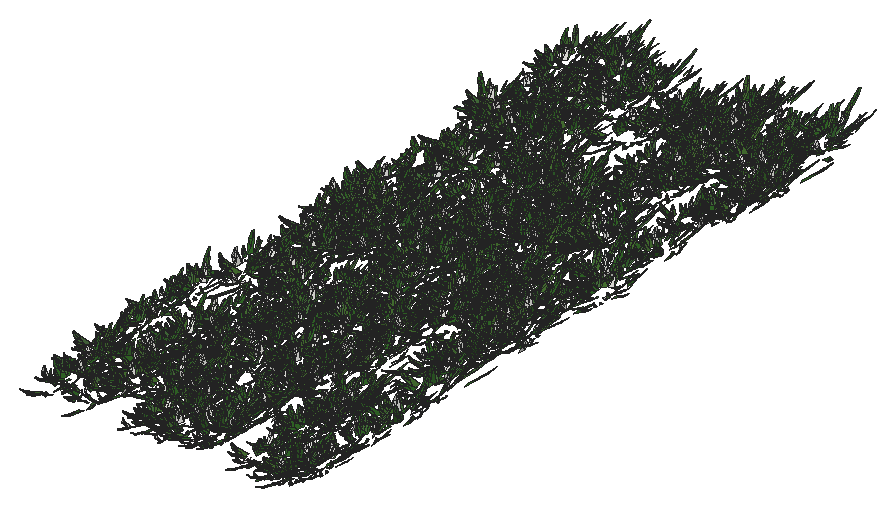
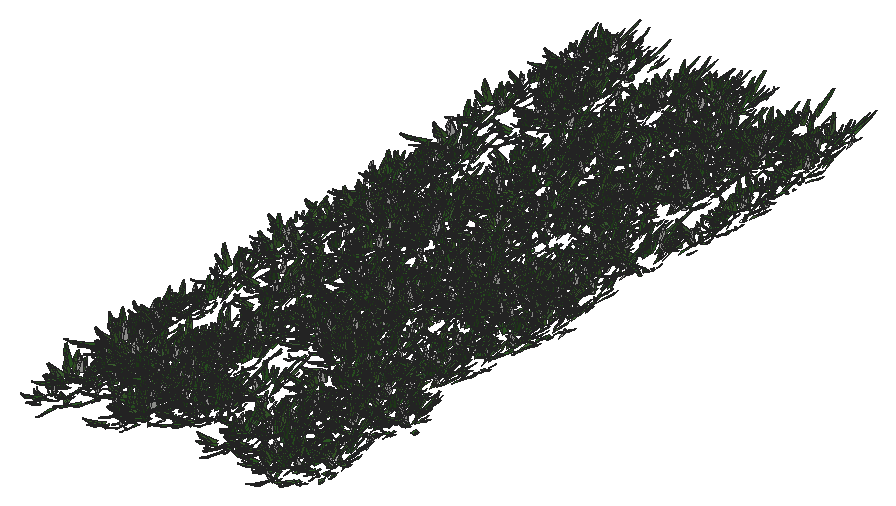
# SketchUp Ruby script. Lengths in inches.
U = 1.inch
M = Sketchup.active_model
def pt(a) = Geom::Point3d.new(a.map { |v| v * U })
def face(e, loops, mat)
  f = e.add_face(loops[0].map { |a| pt(a) })
  loops[1..].each { |l| e.add_face(l.map { |a| pt(a) }).erase! }
  f.material = f.back_material = mat if mat
  f
end
# faces: each face lists its corners as indices into pts; further lists are holes
def faces(e, pts, list, mat = nil) = list.each { |f| face(e, (f[0].is_a?(Array) ? f : [f]).map { |l| l.map { |i| pts[i] } }, mat) }
# xy, xz, yz: faces in a plane at the given z, y or x. An outline is a flat list of corners, or four numbers for a rectangle; further outlines are holes
def ring(l) = l.size == 4 ? [[l[0], l[1]], [l[2], l[1]], [l[2], l[3]], [l[0], l[3]]] : l.each_slice(2).to_a
def flat(e, list, mat, &to3) = list.each { |f| face(e, (f[0].is_a?(Array) ? f : [f]).map { |l| ring(l).map { |u, v| to3.(u, v) } }, mat) }
def xy(e, z, list, mat = nil) = flat(e, list, mat) { |x, y| [x, y, z] }
def xz(e, y, list, mat = nil) = flat(e, list, mat) { |x, z| [x, y, z] }
def yz(e, x, list, mat = nil) = flat(e, list, mat) { |y, z| [x, y, z] }
def lines(e, pts, list) = list.each { |a, b| e.add_line(pt(pts[a]), pt(pts[b])) }
# prism: a flat outline (further loops are holes) pulled along v
def prism(e, loops, v, mat = nil)
  f = face(e, loops, mat); d = Geom::Vector3d.new(v.map { |x| x * U })
  f.pushpull(f.normal.samedirection?(d) ? d.length : -d.length)
end
def box(e, o, s, mat = nil) = prism(e, [[o, [o[0] + s[0], o[1], o[2]], [o[0] + s[0], o[1] + s[1], o[2]], [o[0], o[1] + s[1], o[2]]]], [0, 0, s[2]], mat)
def at(x, y, z, deg = 0) = Geom::Transformation.translation(pt([x, y, z])) * Geom::Transformation.rotation(ORIGIN, Z_AXIS, deg.degrees)
def axes(o, x, y, z) = Geom::Transformation.new([*x, 0, *y, 0, *z, 0, *pt(o).to_a, 1])
def part(name) = M.definitions.add(name)
# library, detail: a bought-in or finely detailed component or shape, given as its bounding box
def library(name, o, s) = part(name).tap { |d| box(d.entities, o, s) }
def detail(e, o, s) = box(e.add_group.entities, o, s)
def put(e, d, t, mat = nil) = e.add_instance(d, t).tap { |i| i.material = mat if mat }
def group(e, t, mat = nil) = e.add_group.tap { |g| g.transformation = t; g.material = mat if mat }.entities
root = M.entities
M.materials.add("Material10").color = [48, 90, 38]
M.materials.add("Material11").color = [68, 110, 48]
M.materials.add("Material12").color = [48, 90, 48]
M.materials.add("Material13").color = [58, 110, 58]
M.materials.add("Material14").color = [58, 90, 38]
M.materials.add("Material15").color = [68, 100, 58]
M.materials.add("Material16").color = [48, 100, 38]
M.materials.add("Material9").color = [68, 110, 58]
c1 = part("grass00")
p = [[-0.6875,0.15,0],[-0.56,0.08,5.52],[-0.04,0.03,2.76],[0.48,-0.02,0],[0.35,-0.02,5.52],[-0.1,-0.14,5.52],
  [-0.12,0.65,8.37],[-0.42,0.65,8.37]]
faces(c1.entities,p,[[0,1,2,3],[3,2,4],[1,5,2],[5,4,2],[1,6,5],[4,5,6],[7,6,1]])
c2 = part("Group16\#1")
put(c2.entities,c1,axes([1.44,-0.61,-0.01],[0.05352,0.12609,0],[-0.10704,0.04543,0.07239],[0.06664,-0.02828,0.11628]),"Material12")
put(c2.entities,c1,axes([0.76,-0.15,-0.01],[0.04676,0.24062,0],[-0.23162,0.04501,0.06642],[0.0652,-0.01267,0.23595]),"Material9")
put(c2.entities,c1,axes([0.79,0.01,-0.01],[-0.00606,0.34651,0],[-0.34381,-0.00602,0.0432],[0.04319,0.00076,0.34386]))
put(c2.entities,c1,axes([1,0.23,-0.01],[-0.07192,0.31144,0],[-0.28722,-0.06632,0.1236],[0.12043,0.02781,0.29478]),"Material11")
put(c2.entities,c1,axes([1.66,0.77,-0.01],[-0.13828,0.29651,0],[-0.21551,-0.1005,0.22471],[0.20365,0.09498,0.23779]),"Material16")
put(c2.entities,c1,axes([0.6875,0.52,-0.01],[-0.18126,0.24051,0],[-0.22746,-0.17142,0.09788],[0.07817,0.05891,0.28481]),"Material11")
put(c2.entities,c1,axes([0.68,0.78,-0.01],[-0.215,0.18688,0],[-0.12385,-0.14248,0.21334],[0.13995,0.16101,0.18878]),"Material9")
put(c2.entities,c1,axes([0.56,1,-0.01],[-0.13756,0.07624,0],[-0.06159,-0.11112,0.0927],[0.04494,0.08108,0.12705]),"Material11")
put(c2.entities,c1,axes([0.2,0.64,-0.01],[-0.23729,0.07254,0],[-0.05711,-0.18681,0.153],[0.04473,0.14632,0.19535]),"Material16")
put(c2.entities,c1,axes([0.0625,0.72,-0.01],[-0.28874,0.02525,0],[-0.02179,-0.24916,0.14647],[0.01276,0.14591,0.25012]),"Material9")
put(c2.entities,c1,axes([-0.08,0.62,-0.01],[-0.34089,-0.04187,0],[0.03255,-0.26504,0.216],[-0.02633,0.21439,0.26703]),"Material16")
put(c2.entities,c1,axes([-0.34,0.98,-0.01],[-0.14314,-0.0493,0],[0.04397,-0.12769,0.06843],[-0.02228,0.0647,0.13505]),"Material16")
put(c2.entities,c1,axes([-0.87,1.45,-0.01],[-0.23488,-0.14114,0],[0.13761,-0.22901,0.06087],[-0.03135,0.05217,0.26717]))
put(c2.entities,c1,axes([-0.72,0.77,-0.01],[-0.14208,-0.13251,0],[0.07209,-0.0773,0.16301],[-0.11118,0.11922,0.1057]),"Material16")
put(c2.entities,c1,axes([-0.62,0.43,-0.01],[-0.14845,-0.21203,0],[0.18654,-0.13061,0.12304],[-0.10079,0.07057,0.22772]),"Material9")
put(c2.entities,c1,axes([-0.68,0.29,-0.01],[-0.13639,-0.32136,0],[0.31723,-0.13464,0.05579],[-0.05136,0.0218,0.34462]),"Material10")
put(c2.entities,c1,axes([-0.64,0.125,-0.01],[-0.0458,-0.23569,0],[0.22124,-0.043,0.08276],[-0.08124,0.01579,0.22538]),"Material13")
put(c2.entities,c1,axes([-1.6,-0.03,-0.01],[0.00576,-0.32897,0],[0.27526,0.00482,0.18018],[-0.18015,-0.00315,0.2753]),"Material11")
put(c2.entities,c1,axes([-1.36,-0.31,-0.01],[0.05718,-0.24765,0],[0.18172,0.04196,0.17267],[-0.16825,-0.03885,0.1865]),"Material16")
put(c2.entities,c1,axes([-1.54,-0.72,-0.01],[0.06537,-0.14017,0],[0.13555,0.06321,0.03939],[-0.0357,-0.01665,0.14956]))
put(c2.entities,c1,axes([-1.19,-0.9,-0.01],[0.09597,-0.12735,0],[0.11214,0.08451,0.07557],[-0.06035,-0.04548,0.14042]),"Material15")
put(c2.entities,c1,axes([-0.47,-0.54,-0.01],[0.11588,-0.10072,0],[0.0618,0.0711,0.12124],[-0.07953,-0.0915,0.0942]))
put(c2.entities,c1,axes([-0.47,-0.84,-0.01],[0.11927,-0.0661,0],[0.06603,0.11913,0.00646],[-0.00313,-0.00565,0.13621]),"Material11")
put(c2.entities,c1,axes([-0.38,-1.24,-0.01],[0.28037,-0.08571,0],[0.0618,0.20215,0.20315],[-0.05939,-0.19428,0.21139]),"Material15")
put(c2.entities,c1,axes([-0.06,-0.66,-0.01],[0.22719,-0.01987,0],[0.01247,0.14255,0.17758],[-0.01547,-0.17691,0.1431]),"Material14")
put(c2.entities,c1,axes([0.11,-0.89,-0.01],[0.14882,0.01828,0],[-0.01058,0.08611,0.12229],[0.01491,-0.12138,0.08676]),"Material12")
put(c2.entities,c1,axes([0.25,-0.72,-0.01],[0.20481,0.07053,0],[-0.06206,0.18022,0.10291],[0.03351,-0.0973,0.1906]),"Material12")
put(c2.entities,c1,axes([0.85,-1.42,-0.01],[0.16481,0.09904,0],[-0.09472,0.15762,0.05616],[0.02893,-0.04814,0.18389]),"Material11")
put(c2.entities,c1,axes([1.01,-1.09,-0.01],[0.21858,0.20385,0],[-0.17495,0.1876,0.15339],[0.10462,-0.11218,0.25652]),"Material16")
put(c2.entities,c1,axes([1.01,-0.71,-0.01],[0.08733,0.12473,0],[-0.06445,0.04512,0.13037],[0.1068,-0.07477,0.07867]),"Material12")
c3 = part("Group15\#1")
put(c3.entities,c2,at(0,0,0))
c4 = part("3darcstudiotree_grass00\#1")
put(c4.entities,c3,at(0,0,0))
put(root,c4,axes([889.11,700.2,12.99],[-2.48857,4.83217,0],[-1.60041,-4.30668,-0.00331],[-0.00933,-0.0251,1.47415]))
put(root,c4,axes([889.45,555.4,12.99],[1.88325,-5.62415,0],[2.2145,3.87465,-0.00025],[0.00077,0.00134,1.45509]))
put(root,c4,axes([890.7,736.79,12.99],[-0.67721,-6.67786,0],[3.30552,-1.75159,-0.01344],[0.04021,-0.02131,1.42931]))
put(root,c4,axes([890.59,527.43,12.99],[1.23508,-6.86534,0],[2.79631,2.62859,-0.00107],[0.00335,0.00315,1.41133]))
put(root,c4,axes([890.07,729.8,12.99],[-1.4659,5.84935,0],[-2.43711,-3.19136,-0.00674],[-0.02223,-0.02911,1.46389]))
put(root,c4,axes([890.29,569.96,12.99],[-1.20792,5.92922,0],[-2.43583,-2.59295,-0.01596],[-0.07323,-0.07796,1.86544]))
put(root,c4,axes([890.73,542.65,12.99],[1.71513,4.00539,0],[-2.12111,4.74593,-0.01876],[-0.05829,0.13042,1.77063]))
put(root,c4,axes([890.87,639.05,12.99],[1.25364,6.64692,0],[-3.14878,3.10311,-0.01792],[-0.0469,0.04622,1.34035]))
put(root,c4,axes([892.5,617.87,12.99],[1.99351,-5.07033,0],[1.82805,3.75557,-0.01288],[0.04404,0.09047,1.54961]))
put(root,c4,axes([893.14,588.73,12.99],[-2.84145,-1.64891,0],[0.79806,-7.18594,-0.00944],[0.0101,-0.09094,1.93444]))
put(root,c4,axes([894.38,665.36,12.99],[-2.41994,-3.76289,0],[1.7496,-5.87931,-0.01911],[0.03346,-0.11243,1.32815]))
put(root,c4,axes([894.17,700.75,12.99],[-2.72326,-0.10093,0],[0.04495,-6.33677,-0.00434],[0.00025,-0.03592,1.37632]))
put(root,c4,axes([894.41,648.52,12.99],[-2.77624,2.98667,0],[-1.27115,-6.17405,-0.0027],[-0.00443,-0.02152,1.57765]))
put(root,c4,axes([894.45,517.39,12.99],[1.92472,-5.7589,0],[2.22303,3.88219,-0.00592],[0.02191,0.03827,1.78738]))
put(root,c4,axes([894.51,633.23,12.99],[-0.10576,6.13122,0],[-3.20045,-0.28845,-0.01193],[-0.05367,-0.00484,1.97773]))
put(root,c4,axes([894.76,507.46,12.99],[0.73477,5.96043,0],[-2.82287,1.81831,-0.02067],[-0.08381,0.05398,1.69495]))
put(root,c4,axes([895.09,711.14,12.99],[2.7201,4.30897,0],[-1.8665,6.15665,-0.01195],[-0.02082,0.06867,1.37528]))
put(root,c4,axes([897.43,681,12.99],[-3.04265,0.35823,0],[-0.15997,-7.0997,-0.00589],[-0.00096,-0.04283,1.35922]))
put(root,c4,axes([898.1,740.56,12.99],[0.23179,-7.22579,0],[2.54694,0.4269,-0.00239],[0.00971,0.00163,1.42634]))
put(root,c4,axes([897,605.72,12.99],[0.62032,6.83292,0],[-2.78217,1.31977,-0.00381],[-0.01551,0.00736,1.62105]))
put(root,c4,axes([898.29,717.4,12.99],[0.42937,-6.32449,0],[2.49768,0.88604,-0.00401],[0.02082,0.00739,1.82024]))
put(root,c4,axes([898.53,618.78,12.99],[0.91628,-5.1494,0],[2.52826,2.35071,-0.0011],[0.00494,0.0046,1.80895]))
put(root,c4,axes([899.48,673.55,12.99],[2.62988,-0.99399,0],[0.55692,7.69933,-0.01648],[0.00872,0.1206,1.51991]))
put(root,c4,axes([899.46,586.64,12.99],[3.4134,1.62353,0],[-0.71308,7.83371,-0.01168],[-0.00692,0.07599,1.39591]))
put(root,c4,axes([900.61,741.23,12.99],[3.44408,-0.25415,0],[0.08694,6.15631,-0.01793],[0.00281,0.19875,1.79317]))
put(root,c4,axes([901.875,703.72,12.99],[0.0032,-6.22666,0],[2.78842,0.0075,-0.01884],[0.07166,0.00019,1.45492]))
put(root,c4,axes([902.12,635.8,12.99],[-2.06596,5.7417,0],[-2.57655,-4.84423,-0.01702],[-0.05495,-0.10332,1.91367]))
put(root,c4,axes([902.1,525.17,12.99],[3.06635,-0.29682,0],[0.12679,6.84401,-0.02002],[0.00349,0.18854,1.69539]))
put(root,c4,axes([903.61,693.23,12.99],[-3.37213,2.17513,0],[-0.90079,-7.29706,-0.00145],[-0.00158,-0.01283,1.8291]))
put(root,c4,axes([903.07,617.46,12.99],[0.95242,7.49428,0],[-2.36141,1.5681,-0.00931],[-0.03611,0.02398,1.3628]))
put(root,c4,axes([904.85,656.18,12.99],[-2.23753,5.4106,0],[-2.13955,-4.62327,-0.01805],[-0.05563,-0.12022,1.71251]))
put(root,c4,axes([905.1875,628.21,12.99],[-2.35532,2.72791,0],[-1.18826,-5.3609,-0.00642],[-0.01064,-0.04801,1.3229]))
put(root,c4,axes([905.07,670.3125,12.99],[-1.67258,4.18596,0],[-2.56199,-5.34901,-0.00484],[-0.0117,-0.02443,1.55938]))
put(root,c4,axes([906.18,644.99,12.99],[-0.78923,-5.50789,0],[3.27099,-2.44906,-0.01545],[0.0482,-0.03609,1.54954]))
put(root,c4,axes([906.22,508.02,12.99],[-0.37406,-5.96975,0],[3.38961,-1.10978,-0.00214],[0.00721,-0.00236,1.59988]))
put(root,c4,axes([905.29,591.09,12.99],[-1.61058,4.76543,0],[-2.42445,-4.28152,-0.01374],[-0.04386,-0.07746,1.69563]))
put(root,c4,axes([905.04,544.16,12.99],[-0.8341,7.12764,0],[-3.0028,-1.83613,-0.00132],[-0.00556,-0.0034,1.858]))
put(root,c4,axes([904.75,618.24,12.99],[2.4007,5.25585,0],[-2.3435,5.59327,-0.01961],[-0.04836,0.11543,1.65716]))
put(root,c4,axes([906.12,532.9,12.99],[-2.70473,0.752,0],[-0.41791,-7.85407,-0.00408],[-0.00182,-0.03415,1.74968]))
put(root,c4,axes([905.07,714.26,12.99],[0.47893,7.6528,0],[-3.19759,1.04564,-0.02596],[-0.07693,0.02516,1.32635]))
put(root,c4,axes([905.23,633.26,12.99],[-0.79693,7.39381,0],[-3.19145,-1.79739,-0.00818],[-0.03214,-0.0181,1.82396]))
put(root,c4,axes([906.84,736.01,12.99],[-2.61883,4.34404,0],[-1.63817,-5.16033,-0.01293],[-0.03819,-0.12029,1.92389]))
put(root,c4,axes([905.92,605.375,12.99],[2.18903,5.14094,0],[-2.299,5.11509,-0.004],[-0.01232,0.02742,1.89371]))
put(root,c4,axes([907.25,563.7,12.99],[-3.06581,1.10697,0],[-0.44175,-6.39285,-0.01239],[-0.00708,-0.10252,1.42361]))
put(root,c4,axes([906.32,552.57,12.99],[3.11337,0.63617,0],[-0.24083,6.15863,-0.01038],[-0.00483,0.12358,1.94021]))
put(root,c4,axes([907.1,694.13,12.99],[1.37515,5.77822,0],[-2.19205,2.7259,-0.01685],[-0.0837,0.10408,1.93576]))
put(root,c4,axes([909.91,733.37,12.99],[-2.98753,-4.03038,0],[1.29962,-5.03369,-0.01139],[0.02516,-0.09747,1.52439]))
put(root,c4,axes([910,522.94,12.99],[-0.33669,-7.20196,0],[2.55571,-0.62431,-0.01446],[0.06571,-0.01605,1.61179]))
put(root,c4,axes([909.59,517.17,12.99],[-2.31485,3.45016,0],[-1.62215,-5.68696,-0.02083],[-0.04485,-0.15725,1.60618]))
put(root,c4,axes([910.25,718.3,12.99],[-2.81133,-1.91296,0],[0.82005,-6.29725,-0.0137],[0.01382,-0.10615,1.39479]))
put(root,c4,axes([910.65,618.72,12.99],[2.31372,-3.04681,0],[1.57401,6.24565,-0.00508],[0.00919,0.03648,1.56982]))
put(root,c4,axes([911.38,580.73,12.99],[1.12741,-7.37052,0],[2.72279,2.17621,-0.01723],[0.05902,0.04717,1.43549]))
put(root,c4,axes([911.67,587.49,12.99],[-2.23921,5.74187,0],[-2.01313,-4.10222,-0.02096],[-0.07106,-0.14481,1.6805]))
put(root,c4,axes([911.47,701.26,12.99],[0.50465,7.81669,0],[-2.42233,0.81716,-0.00575],[-0.02234,0.00754,1.31904]))
put(root,c4,axes([913.04,695.85,12.99],[-2.29321,-5.01245,0],[2.16853,-5.18399,-0.00934],[0.02355,-0.05631,1.57129]))
put(root,c4,axes([913.78,634.85,12.99],[-1.22299,-7.18231,0],[2.62681,-2.33719,-0.00938],[0.03672,-0.03267,1.62403]))
put(root,c4,axes([912.98,618.68,12.99],[2.8573,1.53102,0],[-0.60064,5.85726,-0.007],[-0.00692,0.06752,1.56436]))
put(root,c4,axes([914.47,552.18,12.99],[-2.23311,-2.77512,0],[1.19008,-5.00391,-0.02167],[0.04044,-0.17003,1.33527]))
put(root,c4,axes([914.37,675.69,12.99],[-3.01026,0.37875,0],[-0.16061,-6.6701,-0.00024],[-0.00006,-0.00258,1.85086]))
put(root,c4,axes([914.43,560,12.99],[1.83298,-3.66675,0],[2.06861,5.40332,-0.0129],[0.0274,0.07158,1.39029]))
put(root,c4,axes([914.23,630.17,12.99],[2.78814,-3.17709,0],[1.51248,6.93552,-0.00236],[0.00318,0.01459,1.40454]))
put(root,c4,axes([915.11,723.24,12.99],[-2.92128,-0.49185,0],[0.23367,-7.25198,-0.00991],[0.00283,-0.08779,1.69565]))
put(root,c4,axes([915.56,541.63,12.99],[-0.04494,-6.00078,0],[2.43937,-0.09545,-0.01279],[0.0632,-0.00247,1.65408]))
put(root,c4,axes([915.51,655.5625,12.99],[-0.3518,6.7011,0],[-2.41266,-0.66183,-0.01529],[-0.0761,-0.02088,1.67142]))
put(root,c4,axes([917.06,548.78,12.99],[0.00678,-7.42215,0],[2.83375,0.01353,-0.00952],[0.03556,0.00017,1.45276]))
put(root,c4,axes([917.52,683.87,12.99],[-2.67985,1.60527,0],[-0.6878,-5.99971,-0.00505],[-0.00598,-0.0522,1.74136]))
put(root,c4,axes([918.23,739.07,12.99],[-2.59596,-3.08917,0],[1.33761,-5.87341,-0.02288],[0.04074,-0.17887,1.53217]))
put(root,c4,axes([918.17,639.23,12.99],[2.20522,-2.43928,0],[1.15592,5.46039,-0.0104],[0.01786,0.08439,1.43546]))
put(root,c4,axes([918.18,700.84,12.99],[2.80622,-1.40219,0],[0.61199,6.39972,-0.02018],[0.01648,0.17234,1.50307]))
put(root,c4,axes([919.63,596.52,12.99],[-1.80529,-5.20352,0],[2.41798,-4.38336,-0.01126],[0.02761,-0.05006,1.32461]))
put(root,c4,axes([919.39,573.8,12.99],[-2.50688,-1.35349,0],[0.61589,-5.96052,-0.01801],[0.01504,-0.14556,1.33554]))
put(root,c4,axes([919.06,523.5,12.99],[2.94028,0.786,0],[-0.30241,5.91107,-0.0104],[-0.00633,0.12365,1.87036]))
put(root,c4,axes([919.74,727.91,12.99],[0.86687,7.3097,0],[-2.77933,1.72227,-0.02312],[-0.08493,0.05263,1.50331]))
put(root,c4,axes([921.52,579.83,12.99],[-2.10371,5.02704,0],[-2.26453,-4.95172,-0.01205],[-0.03797,-0.08302,1.87482]))
put(root,c4,axes([922.28,536.86,12.99],[-3.08379,-0.18861,0],[0.08375,-7.15503,-0.01377],[0.00142,-0.12105,1.65227]))
put(root,c4,axes([921.97,639.34,12.99],[-2.36113,3.58907,0],[-1.55051,-5.3299,-0.00165],[-0.00338,-0.0116,1.42237]))
put(root,c4,axes([922.66,559.92,12.99],[-2.39262,-2.63239,0],[1.50419,-7.14383,-0.00367],[0.00536,-0.02548,1.60507]))
put(root,c4,axes([922.375,523.4,12.99],[0.48903,-7.91805,0],[2.87278,0.9271,-0.01886],[0.08181,0.0264,1.74385]))
put(root,c4,axes([921.65,624.83,12.99],[2.7413,0.85853,0],[-0.35937,5.99584,-0.00884],[-0.00625,0.10424,1.89082]))
put(root,c4,axes([923.63,685.9,12.99],[-1.06693,-5.43436,0],[2.89759,-2.97254,-0.01184],[0.03912,-0.04013,1.57815]))
put(root,c4,axes([923.1,667.04,12.99],[1.8875,4.52691,0],[-2.5013,5.4495,-0.0237],[-0.04889,0.10651,1.35093]))
put(root,c4,axes([923.88,573.42,12.99],[2.34934,5.12934,0],[-1.8203,4.35645,-0.00574],[-0.01554,0.0372,1.41814]))
put(root,c4,axes([924.03,675.64,12.99],[1.05033,5.40245,0],[-2.89838,2.94438,-0.00487],[-0.01707,0.01734,1.66894]))
put(root,c4,axes([925.73,610.68,12.99],[2.94911,-3.18283,0],[1.10409,5.3455,-0.01833],[0.02951,0.14285,1.33779]))
put(root,c4,axes([925.68,619.44,12.99],[-1.41119,5.53185,0],[-2.79209,-3.72178,-0.00159],[-0.00501,-0.00668,1.61385]))
put(root,c4,axes([926.09,652.92,12.99],[2.96523,-2.44641,0],[1.02012,6.46078,-0.00463],[0.00681,0.04316,1.7876]))
put(root,c4,axes([927.2,517.72,12.99],[-1.89615,-3.58835,0],[2.01712,-5.5695,-0.02106],[0.04495,-0.12412,1.45262]))
put(root,c4,axes([925.71,595.8,12.99],[0.89643,5.50795,0],[-3.07832,2.61785,-0.01219],[-0.03304,0.0281,1.30286]))
put(root,c4,axes([926.625,568.69,12.99],[-2.24743,4.56313,0],[-1.73205,-4.45747,-0.02123],[-0.05399,-0.13894,1.37003]))
put(root,c4,axes([927.67,681.47,12.99],[0.02696,-5.65578,0],[2.59952,0.06476,-0.01263],[0.06027,0.0015,1.70174]))
put(root,c4,axes([927.79,507.1,12.99],[-1.09532,5.4345,0],[-2.93962,-3.09584,-0.00587],[-0.01769,-0.01863,1.47291]))
put(root,c4,axes([929.6,552.4,12.99],[-2.83178,0.06796,0],[-0.02959,-6.44259,-0.01485],[-0.00066,-0.14283,1.62647]))
put(root,c4,axes([929.53,675.5,12.99],[1.85271,-3.89717,0],[2.18955,5.43899,-0.00074],[0.00191,0.00474,1.68668]))
put(root,c4,axes([929.56,645.76,12.99],[-1.91651,5.84483,0],[-2.53697,-4.3467,-0.01976],[-0.06317,-0.10823,1.7373]))
put(root,c4,axes([929.38,654.48,12.99],[3.13416,-0.63127,0],[0.29357,7.61602,-0.00682],[0.00195,0.05052,1.49182]))
put(root,c4,axes([929.46,711.875,12.99],[3.09979,2.78102,0],[-1.06339,6.19334,-0.00074],[-0.00106,0.00617,1.56313]))
put(root,c4,axes([930.91,662.89,12.99],[-2.96379,-1.31654,0],[0.64355,-7.5701,-0.00093],[0.00055,-0.00644,1.42207]))
put(root,c4,axes([929.72,637.59,12.99],[0.48945,7.25352,0],[-2.6679,0.94067,-0.0058],[-0.02805,0.00989,1.813]))
put(root,c4,axes([930.58,527.34,12.99],[2.3282,-5.17756,0],[1.69862,3.99113,-0.01443],[0.05619,0.13202,1.86565]))
put(root,c4,axes([931.43,587.04,12.99],[-2.96015,-2.26228,0],[0.78218,-5.34781,-0.00172],[0.0023,-0.01572,1.42531]))
put(root,c4,axes([930.4,629.64,12.99],[2.03771,3.36163,0],[-1.92495,6.097,-0.01696],[-0.04044,0.12807,1.8379]))
put(root,c4,axes([930.56,583.26,12.99],[1.16539,4.94873,0],[-2.80252,3.44852,-0.00648],[-0.02198,0.02705,1.68262]))
put(root,c4,axes([932.26,539.33,12.99],[-0.27855,-6.11893,0],[3.41775,-0.81297,-0.00351],[0.011,-0.00262,1.48465]))
put(root,c4,axes([932.26,730.97,12.99],[-1.70025,-5.01216,0],[1.94768,-3.4523,-0.0081],[0.03551,-0.06294,1.87526]))
put(root,c4,axes([933.4,515.09,12.99],[2.37316,-1.80781,0],[0.97129,6.66233,-0.01535],[0.01794,0.12305,1.5577]))
put(root,c4,axes([934.01,581.73,12.99],[-1.31601,6.9375,0],[-2.85459,-2.82946,-0.00354],[-0.01252,-0.01241,1.64409]))
put(root,c4,axes([933.82,730.94,12.99],[2.14771,4.14927,0],[-1.85185,5.00858,-0.00305],[-0.00793,0.02146,1.58836]))
put(root,c4,axes([935.24,681.8,12.99],[-2.86059,4.31841,0],[-1.62827,-5.63589,-0.01955],[-0.03905,-0.13516,1.46911]))
put(root,c4,axes([935.6,506.9,12.99],[-2.32656,1.77433,0],[-0.83368,-5.71198,-0.01591],[-0.02045,-0.14014,1.46774]))
put(root,c4,axes([934.5625,620.78,12.99],[2.2845,4.98317,0],[-2.03439,4.87332,-0.00767],[-0.02399,0.05748,1.8325]))
put(root,c4,axes([935.32,601.03,12.99],[3.0627,-1.98884,0],[0.74033,5.95713,-0.02465],[0.0256,0.20598,1.41248]))
put(root,c4,axes([936.3125,645.22,12.99],[-3.36424,0.55268,0],[-0.2206,-7.01643,-0.01837],[-0.00478,-0.15219,1.53349]))
put(root,c4,axes([935.5,722.8125,12.99],[2.88409,3.07091,0],[-1.14154,5.60196,-0.0112],[-0.02004,0.09836,1.5714]))
put(root,c4,axes([935.96,608.22,12.99],[-1.41458,6.63784,0],[-3.14647,-3.50372,-0.00711],[-0.0179,-0.01993,1.34501]))
put(root,c4,axes([936.4,628.03,12.99],[2.54191,1.16907,0],[-0.49763,5.65361,-0.0192],[-0.01798,0.20428,1.64321]))
put(root,c4,axes([937.84,653.67,12.99],[0.76935,-7.31746,0],[2.65535,1.45879,-0.00397],[0.01891,0.01039,1.83602]))
put(root,c4,axes([938.25,676.45,12.99],[-3.16606,1.84028,0],[-0.63679,-5.72447,-0.01716],[-0.02236,-0.20105,1.87475]))
put(root,c4,axes([937.47,665.03,12.99],[1.50102,6.48692,0],[-2.86017,3.45815,-0.01033],[-0.03141,0.03797,1.52631]))
put(root,c4,axes([939.21,731.34,12.99],[-1.42304,-4.91811,0],[2.32207,-3.51075,-0.00554],[0.0193,-0.02918,1.59445]))
put(root,c4,axes([938.21,558.1875,12.99],[-1.45559,6.6123,0],[-3.0042,-3.45558,-0.00338],[-0.01197,-0.01377,1.82725]))
put(root,c4,axes([939.35,553.78,12.99],[-2.63596,2.31776,0],[-0.89485,-5.31771,-0.01112],[-0.01988,-0.11812,1.70172]))
put(root,c4,axes([940.33,578.25,12.99],[-2.87541,-3.34942,0],[1.56376,-7.01463,-0.02171],[0.03284,-0.1473,1.57387]))
put(root,c4,axes([942.99,704.18,12.99],[-0.73815,-6.09817,0],[2.34694,-1.48441,-0.0133],[0.05599,-0.03541,1.45899]))
put(root,c4,axes([943.47,653.83,12.99],[-2.95268,-3.24899,0],[1.0924,-5.18744,-0.01121],[0.0267,-0.12679,1.89718]))
put(root,c4,axes([942.03,674.33,12.99],[2.74126,3.35097,0],[-1.23861,5.29444,-0.00407],[-0.00847,0.03622,1.59208]))
put(root,c4,axes([942.32,526.2,12.99],[0.30435,7.84756,0],[-2.93148,0.59407,-0.0152],[-0.06026,0.01221,1.60635]))
put(root,c4,axes([943.9,549.51,12.99],[0.17428,-7.43121,0],[3.47978,0.42642,-0.00697],[0.02759,0.00338,1.89407]))
put(root,c4,axes([944.04,727.34,12.99],[2.16406,-4.50203,0],[1.90856,4.7937,-0.00947],[0.02228,0.05597,1.36019]))
put(root,c4,axes([944.56,590.54,12.99],[3.02077,-3.17905,0],[1.07376,5.33129,-0.00355],[0.00674,0.03347,1.60125]))
put(root,c4,axes([944.39,644.24,12.99],[2.44018,1.92258,0],[-0.79244,5.25542,-0.01199],[-0.01544,0.10238,1.31812]))
put(root,c4,axes([944.3,667.48,12.99],[3.19733,2.91365,0],[-0.93386,5.35474,-0.02018],[-0.02989,0.17138,1.38364]))
put(root,c4,axes([944.48,512.16,12.99],[2.50089,5.41721,0],[-2.02485,4.88445,-0.00751],[-0.02321,0.05599,1.8142]))
put(root,c4,axes([946.52,535.89,12.99],[0.74387,-6.89513,0],[2.83321,1.59712,-0.00763],[0.03385,0.01908,1.82848]))
put(root,c4,axes([946.11,742.43,12.99],[2.47185,-3.36887,0],[1.48919,5.70944,-0.01626],[0.03768,0.14447,1.80561]))
put(root,c4,axes([946.96,558.75,12.99],[-1.84488,-3.65611,0],[1.59914,-4.21638,-0.00893],[0.03468,-0.09144,1.98619]))
put(root,c4,axes([946.96,677.29,12.99],[0.87204,-6.97921,0],[2.69034,1.75648,-0.01145],[0.04089,0.0267,1.42532]))
put(root,c4,axes([946.92,617.99,12.99],[1.59063,-4.3766,0],[2.54833,4.83942,-0.00974],[0.0267,0.0507,1.619]))
put(root,c4,axes([947.2,568.5,12.99],[-2.63733,-0.58135,0],[0.31344,-7.43003,-0.0118],[0.00339,-0.08042,1.34216]))
put(root,c4,axes([946.71,587.91,12.99],[3.12558,-2.89481,0],[1.19704,6.75346,-0.01357],[0.02311,0.1304,1.98263]))
put(root,c4,axes([946.46,721.79,12.99],[3.09313,1.18411,0],[-0.53885,7.35502,-0.00046],[-0.00024,0.00328,1.40239]))
put(root,c4,axes([946.7,511.56,12.99],[2.4927,0.72252,0],[-0.3534,6.37077,-0.01144],[-0.00635,0.11454,1.7012]))
put(root,c4,axes([948.47,521.84,12.99],[-0.68736,-7.44146,0],[2.79674,-1.34984,-0.00703],[0.02647,-0.01277,1.50812]))
put(root,c4,axes([948.62,554.26,12.99],[-1.59877,-4.61804,0],[2.30563,-4.17084,-0.00813],[0.02088,-0.03778,1.32168]))
put(root,c4,axes([948.68,689.25,12.99],[-1.68888,-4.17629,0],[2.05191,-4.33581,-0.01026],[0.03403,-0.07191,1.73127]))
put(root,c4,axes([947.4375,626.67,12.99],[1.88136,4.81447,0],[-1.87849,3.83563,-0.01423],[-0.05616,0.11467,1.82816]))
put(root,c4,axes([947.58,643.96,12.99],[1.27105,5.37471,0],[-2.64381,3.26695,-0.00296],[-0.00981,0.01212,1.55057]))
put(root,c4,axes([948.18,611.5625,12.99],[-1.73912,6.09796,0],[-2.34777,-3.49868,-0.00573],[-0.02047,-0.0305,1.63969]))
put(root,c4,axes([949.73,610.24,12.99],[-2.21423,-4.3499,0],[1.80597,-4.80351,-0.00129],[0.00324,-0.00863,1.46122]))
put(root,c4,axes([950.32,746.07,12.99],[-1.51861,-5.47127,0],[2.20981,-3.20492,-0.00968],[0.03949,-0.05727,1.73508]))
put(root,c4,axes([950.43,727.69,12.99],[-0.45735,-5.73272,0],[3.34661,-1.39508,-0.01194],[0.04005,-0.01669,1.59034]))
put(root,c4,axes([950.93,579.73,12.99],[-0.93143,-5.68237,0],[3.27843,-2.80798,-0.00645],[0.01655,-0.01418,1.31612]))
put(root,c4,axes([950.52,689.26,12.99],[-2.29297,4.5898,0],[-1.76278,-4.60159,-0.00238],[-0.00814,-0.02124,1.90825]))
put(root,c4,axes([950.33,717.56,12.99],[0.21322,7.00042,0],[-2.72772,0.43411,-0.01352],[-0.05389,0.00858,1.49862]))
put(root,c4,axes([951.67,602.03,12.99],[-0.12785,-5.65203,0],[3.34159,-0.39496,-0.00424],[0.01462,-0.00173,1.58408]))
put(root,c4,axes([951.875,736.31,12.99],[-3.36007,-2.11521,0],[0.8628,-7.16162,-0.00177],[0.00183,-0.0152,1.73275]))
put(root,c4,axes([951.17,703.77,12.99],[-1.45457,4.6252,0],[-2.43777,-4.00593,-0.0015],[-0.004,-0.00657,1.35234]))
put(root,c4,axes([952.51,552.02,12.99],[-3.22802,-2.971,0],[1.21199,-6.88078,-0.01703],[0.02347,-0.13326,1.64249]))
put(root,c4,axes([951.58,711.71,12.99],[-0.59602,6.68561,0],[-3.08046,-1.43497,-0.00834],[-0.03279,-0.01527,1.72954]))
put(root,c4,axes([951.89,653.05,12.99],[0.79785,6.41123,0],[-3.26339,2.12204,-0.01266],[-0.04487,0.02917,1.71446]))
put(root,c4,axes([954.15,636.15,12.99],[1.24442,-6.08411,0],[2.88578,3.08417,-0.01397],[0.05041,0.05388,1.74087]))
put(root,c4,axes([955,570.09,12.99],[-2.65349,-0.32806,0],[0.13894,-5.87228,-0.00522],[0.00112,-0.04733,1.40302]))
put(root,c4,axes([955.79,626.05,12.99],[-2.07772,-3.24978,0],[1.61153,-5.38367,-0.01797],[0.0355,-0.1186,1.36964]))
put(root,c4,axes([955.89,700.43,12.99],[1.51767,-4.91301,0],[2.24959,3.63109,-0.00946],[0.03305,0.05335,1.61646]))
put(root,c4,axes([955.69,722.01,12.99],[2.57538,0.85446,0],[-0.47057,7.411,-0.0224],[-0.01015,0.15978,1.41716]))
put(root,c4,axes([956.1,607.29,12.99],[1.54629,4.41449,0],[-2.12387,3.88725,-0.01526],[-0.06231,0.11405,1.9517]))
put(root,c4,axes([958.38,673.92,12.99],[-2.60003,-2.65843,0],[1.05909,-5.41243,-0.00732],[0.01412,-0.07215,1.68082]))
put(root,c4,axes([958.81,618.63,12.99],[-0.6227,-5.38828,0],[3.2109,-1.93892,-0.01354],[0.05475,-0.03306,1.90468]))
put(root,c4,axes([958.71,663,12.99],[-2.09584,4.06138,0],[-1.84422,-4.97281,-0.0209],[-0.05115,-0.13793,1.48072]))
put(root,c4,axes([958.21,596.22,12.99],[2.70049,4.4771,0],[-1.55785,4.90995,-0.01189],[-0.02884,0.09088,1.50367]))
put(root,c4,axes([958.89,658.01,12.99],[-1.84968,4.45285,0],[-2.48734,-5.39883,-0.01749],[-0.04827,-0.10477,1.7911]))
put(root,c4,axes([959.61,719.8,12.99],[0.75072,-5.96506,0],[3.10012,2.03866,-0.0144],[0.05652,0.03717,1.80693]))
put(root,c4,axes([958.42,626.28,12.99],[2.53891,4.39772,0],[-1.91654,5.78151,-0.0181],[-0.03384,0.10207,1.34745]))
put(root,c4,axes([958.68,694.66,12.99],[0.62463,6.58281,0],[-2.38185,1.18094,-0.00976],[-0.04638,0.02299,1.62508]))
put(root,c4,axes([960.19,536.7,12.99],[0.08916,-6.8124,0],[3.09273,0.2115,-0.01737],[0.06332,0.00433,1.54781]))
put(root,c4,axes([960.49,709.13,12.99],[-2.95212,4.02036,0],[-1.56398,-6.00074,-0.00882],[-0.01536,-0.05892,1.42641]))
put(root,c4,axes([962.72,639.01,12.99],[-3.04064,-1.62133,0],[0.56924,-5.57825,-0.01564],[0.01416,-0.13875,1.3694]))
put(root,c4,axes([963.15,616.83,12.99],[-2.7685,-2.32333,0],[0.95425,-5.94156,-0.02574],[0.03234,-0.20136,1.38465]))
put(root,c4,axes([963.76,664.44,12.99],[-3.23027,-1.88448,0],[0.60124,-5.3852,-0.00096],[0.00112,-0.01006,1.58162]))
put(root,c4,axes([963.96,552.91,12.99],[-2.95191,-2.11458,0],[0.79093,-5.76926,-0.00157],[0.00178,-0.01301,1.37913]))
put(root,c4,axes([964.29,723.6875,12.99],[0.98009,-6.92855,0],[2.57983,1.90686,-0.02554],[0.09177,0.06783,1.40467]))
put(root,c4,axes([963.47,738.65,12.99],[1.91293,4.81392,0],[-2.04314,4.24231,-0.01914],[-0.05312,0.1103,1.41957]))
put(root,c4,axes([963.35,524.36,12.99],[1.07465,6.4366,0],[-3.03598,2.64858,-0.00597],[-0.02279,0.01988,1.82255]))
put(root,c4,axes([963.78,508.44,12.99],[2.69038,1.72605,0],[-0.66114,5.38465,-0.00495],[-0.00554,0.0451,1.38942]))
put(root,c4,axes([964.29,542.9,12.99],[-1.3689,4.62239,0],[-2.43446,-3.76716,-0.00267],[-0.00888,-0.01373,1.62102]))
put(root,c4,axes([964.34,532.56,12.99],[2.42602,3.51267,0],[-1.81681,6.55647,-0.01012],[-0.01844,0.06656,1.58691]))
put(root,c4,axes([967.38,579.57,12.99],[-2.1204,-3.10851,0],[1.44005,-5.13273,-0.01822],[0.04294,-0.15305,1.59761]))
put(root,c4,axes([967.2,539.93,12.99],[-2.66068,3.18829,0],[-1.12977,-4.92638,-0.02232],[-0.04937,-0.21529,1.59039]))
put(root,c4,axes([966.19,600.56,12.99],[1.09861,5.48105,0],[-2.93064,3.06936,-0.00338],[-0.01071,0.01121,1.53978]))
put(root,c4,axes([966.73,721.26,12.99],[3.09142,-0.99385,0],[0.46979,7.6357,-0.01318],[0.00788,0.12808,1.98636]))
put(root,c4,axes([967.66,616.79,12.99],[1.21093,-7.16225,0],[2.80651,2.47937,-0.011],[0.03697,0.03266,1.48653]))
put(root,c4,axes([968.73,536.61,12.99],[-1.18821,-4.89962,0],[2.9226,-3.70342,-0.00731],[0.02758,-0.03495,1.97847]))
put(root,c4,axes([968.73,728.88,12.99],[-1.91326,-5.66309,0],[2.3144,-4.08567,-0.00917],[0.02902,-0.05124,1.60374]))
put(root,c4,axes([968.75,609.1,12.99],[-2.45984,1.22799,0],[-0.55934,-5.85451,-0.01018],[-0.00821,-0.08595,1.35975]))
put(root,c4,axes([972.11,684.41,12.99],[-1.40819,-5.30727,0],[2.41766,-3.35191,-0.01057],[0.04317,-0.05985,1.85267]))
put(root,c4,axes([971.87,617.62,12.99],[-2.82213,0.67884,0],[-0.36704,-7.97304,-0.00853],[-0.00321,-0.06983,1.7318]))
put(root,c4,axes([971.68,507.97,12.99],[1.6993,-4.1303,0],[2.09234,4.49808,-0.02136],[0.06403,0.13765,1.62144]))
put(root,c4,axes([972.6,588.51,12.99],[-2.91912,-1.23779,0],[0.55217,-6.80424,-0.00704],[0.00576,-0.07098,1.86241]))
put(root,c4,axes([971.57,642.91,12.99],[-0.63556,7.1999,0],[-2.59928,-1.19891,-0.00527],[-0.02725,-0.01257,1.91768]))
put(root,c4,axes([971.8,581.2,12.99],[1.33466,4.81368,0],[-2.90353,4.20653,-0.01772],[-0.04376,0.06339,1.37883]))
put(root,c4,axes([972.62,745.98,12.99],[-0.51246,7.31119,0],[-3.18925,-1.16805,-0.01053],[-0.0368,-0.01348,1.56894]))
put(root,c4,axes([973.14,596.18,12.99],[-1.81597,5.33653,0],[-2.57747,-4.58297,-0.01031],[-0.03029,-0.05385,1.66779]))
put(root,c4,axes([974.55,741.03,12.99],[2.38406,-5.3346,0],[2.2562,5.26863,-0.00616],[0.01614,0.03769,1.65812]))
put(root,c4,axes([975.11,648.71,12.99],[1.71389,-5.3153,0],[2.76675,4.66155,-0.00987],[0.0321,0.05408,1.9048]))
put(root,c4,axes([974.66,625.83,12.99],[2.83528,-2.77005,0],[1.11298,5.95252,-0.01454],[0.01918,0.10256,1.30369]))
put(root,c4,axes([975.36,713.35,12.99],[-2.49642,0.4038,0],[-0.22228,-7.18029,-0.01026],[-0.00285,-0.09212,1.70108]))
put(root,c4,axes([975.21,512.71,12.99],[3.41778,1.78556,0],[-0.61839,6.18495,-0.00333],[-0.00267,0.02669,1.36941]))
put(root,c4,axes([976.08,607.93,12.99],[-2.26095,4.6192,0],[-2.05949,-5.26731,-0.02716],[-0.05664,-0.14485,1.32671]))
put(root,c4,axes([976.91,597.62,12.99],[-1.57495,-7.13241,0],[2.82848,-3.26355,-0.02075],[0.07135,-0.08233,1.67433]))
put(root,c4,axes([976.03,718.3125,12.99],[2.60336,-4.49517,0],[1.53534,4.64619,-0.01203],[0.03979,0.12041,1.91781]))
put(root,c4,axes([976.78,666.78,12.99],[-2.91526,1.469,0],[-0.5875,-6.09214,-0.01188],[-0.01364,-0.14143,1.99665]))
put(root,c4,axes([975.92,692.81,12.99],[0.63511,6.83364,0],[-2.71779,1.31983,-0.01067],[-0.05012,0.02434,1.82972]))
put(root,c4,axes([976.46,507.39,12.99],[2.75237,1.85251,0],[-0.77986,6.05435,-0.01058],[-0.01212,0.09409,1.53588]))
put(root,c4,axes([976.79,699.17,12.99],[2.37835,1.48296,0],[-0.74441,6.23823,-0.00322],[-0.00434,0.0364,1.99197]))
put(root,c4,axes([977.06,567.4,12.99],[3.25727,1.28012,0],[-0.54305,7.22023,-0.00744],[-0.00527,0.07001,1.83611]))
put(root,c4,axes([978.84,698.91,12.99],[-2.40986,-0.93195,0],[0.4275,-5.77625,-0.02254],[0.01491,-0.20145,1.39425]))
put(root,c4,axes([979.06,549.23,12.99],[-2.66189,1.35875,0],[-0.67319,-6.89112,-0.00123],[-0.00126,-0.01287,1.99006]))
put(root,c4,axes([978.43,713.4375,12.99],[3.11841,2.38332,0],[-0.85814,5.86695,-0.01696],[-0.02625,0.17944,1.81122]))
put(root,c4,axes([978.96,532.47,12.99],[1.40608,5.17146,0],[-2.22318,3.15847,-0.00184],[-0.00698,0.00991,1.60144]))
put(root,c4,axes([979.27,638.25,12.99],[-0.71596,5.66819,0],[-3.08403,-2.03549,-0.01983],[-0.06254,-0.04128,1.44555]))
put(root,c4,axes([979.64,515.43,12.99],[-1.33484,5.26758,0],[-2.22521,-2.94641,-0.02138],[-0.08569,-0.11347,1.63406]))
